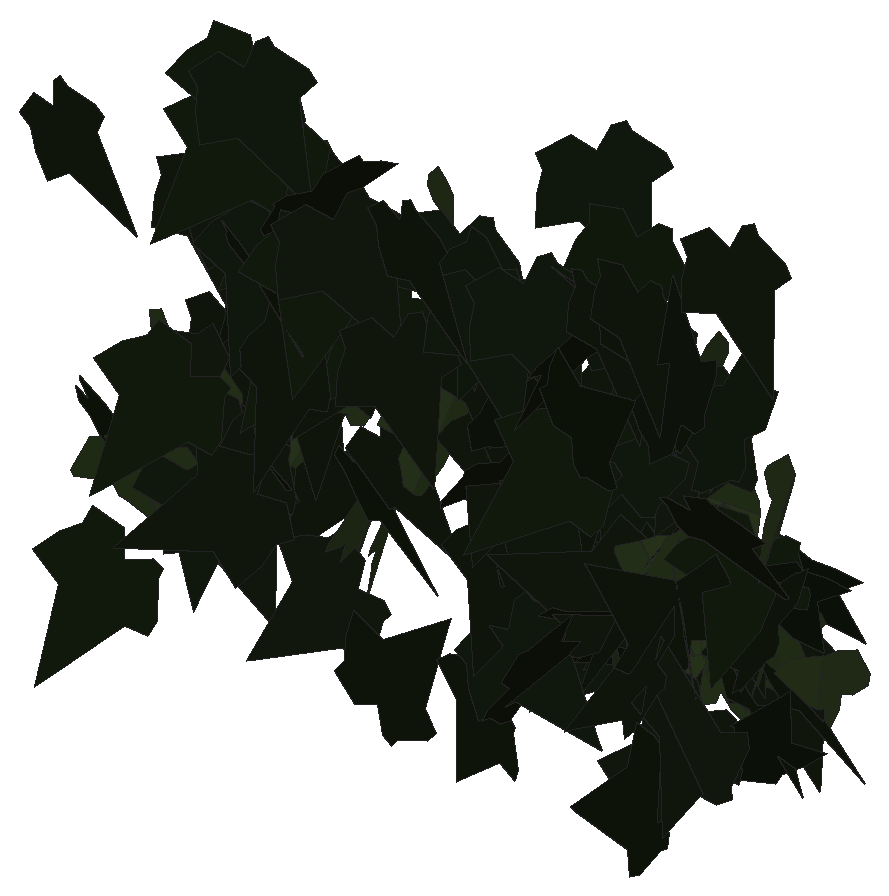
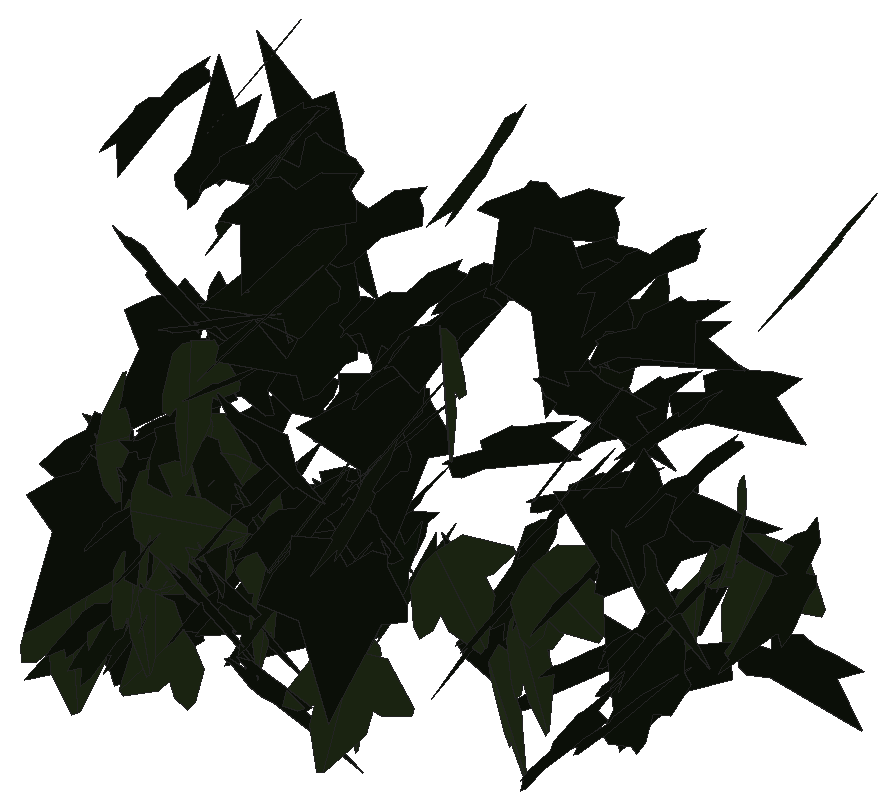
# SketchUp Ruby script. Lengths in inches.
U = 1.inch
M = Sketchup.active_model
def pt(a) = Geom::Point3d.new(a.map { |v| v * U })
def face(e, loops, mat)
  f = e.add_face(loops[0].map { |a| pt(a) })
  loops[1..].each { |l| e.add_face(l.map { |a| pt(a) }).erase! }
  f.material = f.back_material = mat if mat
  f
end
# faces: each face lists its corners as indices into pts; further lists are holes
def faces(e, pts, list, mat = nil) = list.each { |f| face(e, (f[0].is_a?(Array) ? f : [f]).map { |l| l.map { |i| pts[i] } }, mat) }
# xy, xz, yz: faces in a plane at the given z, y or x. An outline is a flat list of corners, or four numbers for a rectangle; further outlines are holes
def ring(l) = l.size == 4 ? [[l[0], l[1]], [l[2], l[1]], [l[2], l[3]], [l[0], l[3]]] : l.each_slice(2).to_a
def flat(e, list, mat, &to3) = list.each { |f| face(e, (f[0].is_a?(Array) ? f : [f]).map { |l| ring(l).map { |u, v| to3.(u, v) } }, mat) }
def xy(e, z, list, mat = nil) = flat(e, list, mat) { |x, y| [x, y, z] }
def xz(e, y, list, mat = nil) = flat(e, list, mat) { |x, z| [x, y, z] }
def yz(e, x, list, mat = nil) = flat(e, list, mat) { |y, z| [x, y, z] }
def lines(e, pts, list) = list.each { |a, b| e.add_line(pt(pts[a]), pt(pts[b])) }
# prism: a flat outline (further loops are holes) pulled along v
def prism(e, loops, v, mat = nil)
  f = face(e, loops, mat); d = Geom::Vector3d.new(v.map { |x| x * U })
  f.pushpull(f.normal.samedirection?(d) ? d.length : -d.length)
end
def box(e, o, s, mat = nil) = prism(e, [[o, [o[0] + s[0], o[1], o[2]], [o[0] + s[0], o[1] + s[1], o[2]], [o[0], o[1] + s[1], o[2]]]], [0, 0, s[2]], mat)
def at(x, y, z, deg = 0) = Geom::Transformation.translation(pt([x, y, z])) * Geom::Transformation.rotation(ORIGIN, Z_AXIS, deg.degrees)
def axes(o, x, y, z) = Geom::Transformation.new([*x, 0, *y, 0, *z, 0, *pt(o).to_a, 1])
def part(name) = M.definitions.add(name)
# library, detail: a bought-in or finely detailed component or shape, given as its bounding box
def library(name, o, s) = part(name).tap { |d| box(d.entities, o, s) }
def detail(e, o, s) = box(e.add_group.entities, o, s)
def put(e, d, t, mat = nil) = e.add_instance(d, t).tap { |i| i.material = mat if mat }
def group(e, t, mat = nil) = e.add_group.tap { |g| g.transformation = t; g.material = mat if mat }.entities
root = M.entities
M.materials.add("efeu1").color = [18, 25, 13]
M.materials.add("efeu2").color = [43, 57, 29]
c1 = part("ivyleaf_9")
p = [[1.54,2.16,1.25],[1.36,2.04,1.19],[-0.21,0.99,0.68],[-0.71,1.11,0.82],[-0.85,0.86,0.67],[-0.8,0.17,0.21],
  [-0.9,-0.01,0.1],[-0.67,-0.16,-0.02],[-0.08,-0.08,-0.05],[-0.03,-0.6,-0.4],[0.65,-0.88,-0.66],[0.83,-0.6,-0.49],
  [1.29,-0.42,-0.43],[1.8125,-0.07,-0.26],[1.21,0.44,0.15]]
faces(c1.entities,p,[[0,1,2,3,4,5,6,7,8,9,10,11,12,13,14]],"efeu1")
c2 = part("ivyleaf_10")
p = [[0,0.5,-0.03],[-0.0625,2.02,-0.43],[-0.19,2.01,-0.46],[-0.54,1.05,-0.29],[-0.52,0.625,-0.18],[-0.83,0.76,-0.28],
  [-1.16,0.64,-0.33],[-1.15,0.33,-0.24],[-0.77,-0.39,0.02],[-0.3,-0.51,0.16],[0.04,-0.48,0.23],[-0.02,2.01,-0.4375],
  [-0.06,2.01,-0.43],[0.04,-0.49,0.23],[0.67,-0.49,0.14],[1.38,0.36,-0.2],[1.375,0.51,-0.24],[0.81,0.65,-0.19],
  [0.62,0.59,-0.15],[0.6,1.09,-0.28],[0.5,1.23,-0.31]]
faces(c2.entities,p,[[0,1,2,3,4,5,6,7,8,9,10],[11,12,0,13,14,15,16,17,18,19,20]],"efeu2")
put(root,c1,axes([37.94,218.92,253.93],[0.31107,-0.3532,-0.16877],[-0.06359,0.16711,-0.46694],[0.38626,0.31196,0.05905]))
put(root,c1,axes([37.98,219.44,250.43],[0.43291,-0.22548,-0.10839],[-0.09049,0.06083,-0.48797],[0.23324,0.44211,0.01186]))
put(root,c1,axes([38.08,221.1,252.23],[0.08499,-0.48929,-0.05807],[0.02582,0.06327,-0.49531],[0.49205,0.0812,0.03603]))
put(root,c1,axes([38.19,221.3,250.65],[0.18802,-0.45638,-0.07977],[-0.02468,0.0761,-0.49356],[0.46264,0.18954,0.00609]))
put(root,c1,axes([38.63,221.29,251.3125],[-0.40733,0.25168,-0.14401],[0.11208,-0.09236,-0.47844],[-0.26743,-0.42205,0.01883]))
put(root,c2,axes([38.38,219.93,251.125],[-0.20143,0.40317,-0.21651],[0.07165,-0.20586,-0.44999],[-0.45199,-0.21231,0.02516]))
put(root,c1,axes([38.6875,218.96,249.12],[-0.45267,-0.21002,-0.0313],[0.029,0.01186,-0.49902],[0.21035,-0.4536,0.00144]))
put(root,c2,axes([38.6,219.23,250.24],[-0.4384,-0.19936,-0.13439],[0.11846,0.06411,-0.48152],[0.20922,-0.45403,-0.00898]))
put(root,c2,axes([38.61,220.32,250.48],[-0.06607,0.477,-0.13456],[0.01467,-0.13381,-0.48154],[-0.4954,-0.06758,0.00369]))
put(root,c1,axes([38.65,221.11,253.67],[-0.21464,-0.44733,0.06182],[-0.00726,-0.06502,-0.4957],[0.45153,-0.2137,0.02141]))
put(root,c1,axes([38.33,221.52,251.59],[0.24057,-0.21984,0.3792],[0.28084,-0.2548,-0.32589],[0.33653,0.36979,0.00089]))
put(root,c1,axes([38.55,220.71,252.5],[0.26925,-0.33348,-0.25747],[-0.01902,0.29563,-0.40279],[0.42088,0.2267,0.14651]))
put(root,c1,axes([38.76,221.4,249.4],[-0.16154,-0.40828,0.23918],[0.0026,-0.2535,-0.43097],[0.47318,-0.138,0.08402]))
put(root,c1,axes([38.97,220.6875,253.22],[-0.36194,-0.31409,0.14265],[-0.07413,-0.13111,-0.47678],[0.3369,-0.36628,0.04834]))
put(root,c1,axes([39.17,219.76,250.9],[-0.4859,-0.00921,0.11755],[-0.11753,-0.00238,-0.48598],[0.00951,-0.49991,0.00015]))
put(root,c1,axes([38.56,221.06,249.46],[0.06355,-0.2335,0.43754],[0.27744,-0.3489,-0.22649],[0.41108,0.27157,0.08522]))
put(root,c1,axes([38.93,220.3,249.48],[-0.0009,-0.42571,-0.26223],[0.04803,0.26095,-0.42379],[0.49769,-0.02595,0.04042]))
put(root,c1,axes([39.09,221.9,249.2],[-0.08746,-0.40199,0.28418],[-0.03472,-0.28287,-0.41083],[0.49107,-0.0916,0.02157]))
put(root,c1,axes([39.13,220.49,249.93],[-0.11468,-0.45361,0.17632],[-0.02204,-0.17613,-0.46743],[0.48617,-0.11498,0.02041]))
put(root,c1,axes([38.99,221.59,252.53],[0.22043,-0.44736,-0.03585],[-0.01789,0.03115,-0.49871],[0.44843,0.22114,-0.00227]))
put(root,c1,axes([39.1,219.81,249.96],[-0.04756,-0.49632,0.03742],[0.00435,-0.038,-0.49853],[0.49771,-0.04709,0.00793]))
put(root,c1,axes([39.04,220.5,254.05],[0.10646,-0.42962,-0.23258],[0.0347,0.24409,-0.43499],[0.4873,0.07647,0.08179]))
put(root,c1,axes([39.46,221.11,252.71],[-0.48139,-0.13469,0.01123],[-0.00951,-0.0077,-0.49985],[0.13482,-0.48146,0.00485]))
put(root,c1,axes([39.36,220.53,252.23],[-0.13388,-0.46702,0.11818],[-0.00787,-0.12053,-0.48519],[0.48168,-0.13177,0.02492]))
put(root,c1,axes([39.64,218.79,251.59],[-0.36767,-0.32625,0.09154],[-0.07677,-0.05137,-0.49139],[0.33004,-0.37539,-0.01232]))
put(root,c1,axes([39.34,221.17,250.65],[0.05622,-0.48751,0.0958],[0.01464,-0.09475,-0.49072],[0.49661,0.05798,0.00362]))
put(root,c2,axes([39.66,221.27,250.56],[-0.18255,-0.3388,0.3192],[0.00515,-0.34432,-0.36252],[0.46546,-0.12907,0.1292]))
put(root,c1,axes([39.71,220.84,251.375],[-0.31245,-0.36813,0.12982],[0.01201,-0.17527,-0.46812],[0.39017,-0.28941,0.11837]))
put(root,c1,axes([40.02,219.35,250.17],[-0.03955,-0.18419,-0.46315],[-0.0133,-0.46405,0.18568],[-0.49826,0.02701,0.03181]))
put(root,c1,axes([39.85,221.01,251.1],[-0.08184,-0.3862,0.30684],[-0.02083,-0.30805,-0.39328],[0.49282,-0.07716,0.03434]))
put(root,c1,axes([39.78,219.77,252.4],[0.14237,-0.32323,0.35391],[0.20636,-0.29189,-0.34959],[0.43261,0.24561,0.05029]))
put(root,c1,axes([40.19,220.125,253.3],[0.1405,0.47912,0.02647],[0.00961,0.02477,-0.49929],[-0.47976,0.14081,-0.00225]))
put(root,c2,axes([40.18,221.35,249.28],[0.24768,-0.43322,0.03116],[0.01107,-0.02957,-0.499],[0.4342,0.24788,-0.00506]))
put(root,c2,axes([40.29,220.84,249.54],[0.11401,-0.48629,0.02298],[-0.00139,-0.02393,-0.49943],[0.48683,0.11382,-0.00681]))
put(root,c1,axes([40.42,220.43,248.78],[-0.28231,-0.27839,0.30463],[-0.10902,-0.30567,-0.38037],[0.39801,-0.28119,0.11189]))
put(root,c1,axes([40.43,219.54,251.86],[-0.43205,-0.05215,-0.24619],[0.24228,0.04612,-0.43494],[0.06808,-0.49513,-0.01458]))
put(root,c1,axes([40.49,221.18,251.71],[-0.31409,-0.35015,0.16955],[-0.05255,-0.17773,-0.46438],[0.38547,-0.30953,0.07484]))
put(root,c1,axes([40.28,221.1,250.09],[0.28149,-0.3472,-0.22409],[-0.09424,0.21005,-0.44384],[0.40235,0.29211,0.05281]))
put(root,c2,axes([40.71,221.52,250.4],[-0.15062,-0.42481,0.21646],[0.01978,-0.23238,-0.44228],[0.47636,-0.12466,0.08681]))
put(root,c1,axes([40.4375,220.5,250.12],[0.39536,-0.30238,-0.04748],[-0.03622,0.03081,-0.49773],[0.30394,0.39701,0.00246]))
put(root,c2,axes([40.81,221.4,252.75],[0.33334,-0.30971,-0.20729],[-0.06296,0.22732,-0.44087],[0.36732,0.32001,0.11255]))
put(root,c1,axes([40.74,219.66,253],[-0.2313,-0.44035,-0.05088],[0.0258,0.04392,-0.4974],[0.44253,-0.23272,0.00241]))
put(root,c1,axes([41.01,219.4375,253.51],[-0.05242,-0.3479,-0.35527],[0.1452,0.33096,-0.34552],[0.47557,-0.13939,0.06633]))
put(root,c1,axes([41.28,221.03,252.73],[-0.00397,-0.49095,-0.09464],[0.00418,0.0946,-0.49095],[0.49997,-0.00469,0.00335]))
put(root,c1,axes([41.4375,219.59,248.28],[-0.18447,0.11953,0.44909],[0.34298,-0.29102,0.21834],[0.31359,0.38861,0.02538]))
put(root,c1,axes([41.51,221.73,251.1],[0.35378,-0.32628,-0.1356],[-0.09822,0.09351,-0.48126],[0.33941,0.36715,0.00207]))
put(root,c1,axes([41.78,221.77,250.15],[0.31682,0.32271,-0.21326],[-0.15115,-0.15047,-0.45223],[-0.35606,0.35102,0.00221]))
put(root,c1,axes([41.64,221.24,252.29],[-0.07125,-0.4399,0.22675],[-0.02798,-0.22514,-0.44557],[0.49411,-0.07618,0.00746]))
put(root,c1,axes([41.6,220.97,251.55],[0.15039,-0.47232,0.06552],[0.01618,-0.0636,-0.49567],[0.47657,0.15121,-0.00385]))
put(root,c1,axes([41.77,219.4,252.47],[0.04234,-0.45452,-0.20401],[-0.01739,0.20327,-0.45648],[0.4979,0.04575,0.00141]))
put(root,c2,axes([41.92,221.55,248.84],[-0.35045,-0.34055,-0.1059],[0.12979,0.0165,-0.48258],[0.33217,-0.36573,0.07684]))
put(root,c1,axes([41.73,221.2,249.53],[0.01049,-0.23126,0.44318],[0.10511,-0.43235,-0.2281],[0.48871,0.09795,0.03954]))
put(root,c1,axes([41.79,219.51,253.74],[0.29994,-0.39767,-0.0435],[-0.02218,0.03775,-0.49808],[0.39943,0.30072,0.00501]))
put(root,c1,axes([42.03,220.51,252.59],[0.02693,-0.47627,-0.14979],[0.01673,0.15079,-0.47643],[0.49899,0.02065,0.02406]))
put(root,c1,axes([42.15,220.49,251.04],[0.04594,0.07772,0.49178],[0.28341,0.40197,-0.09],[-0.40935,0.28702,-0.00712]))
put(root,c1,axes([42.16,220.66,250.82],[-0.07819,-0.43823,0.22769],[0.0357,-0.23494,-0.43992],[0.49256,-0.05254,0.06802]))
put(root,c2,axes([42.39,220.97,248.75],[0.15018,-0.46691,-0.09714],[-0.0137,0.09758,-0.49019],[0.47672,0.1499,0.01652]))
put(root,c1,axes([42.48,220.18,251.04],[0.07405,0.4903,-0.06422],[-0.01235,-0.06308,-0.49585],[-0.49433,0.07502,0.00276]))
put(root,c1,axes([42.78,221.86,251.26],[-0.46361,0.08666,-0.16601],[-0.16675,0.01069,0.47125],[0.08522,0.49232,0.01899]))
put(root,c1,axes([42.52,220.83,250.17],[-0.43007,-0.07254,-0.24449],[0.23876,0.05394,-0.43599],[0.08963,-0.49176,-0.01176]))
put(root,c1,axes([42.3,221.67,250.53],[0.09053,-0.44675,0.20548],[0.03452,-0.20264,-0.45579],[0.49052,0.09671,-0.00585]))
put(root,c1,axes([42.4,220.36,249.79],[-0.04837,-0.42669,0.25611],[0.021,-0.25884,-0.42727],[0.49721,-0.03058,0.04296]))
put(root,c1,axes([42.86,221.82,248.65],[-0.49701,0.05229,0.01578],[-0.01814,-0.02179,-0.4992],[-0.05152,-0.49678,0.02356]))
put(root,c1,axes([42.59,221.5,250.4375],[0.02454,-0.48577,-0.11588],[-0.01917,0.11502,-0.48621],[0.49903,0.02831,-0.01298]))
put(root,c1,axes([42.625,221.5,253.9375],[-0.03978,-0.38436,-0.31731],[0.02871,0.31602,-0.3864],[0.49759,-0.04896,-0.00307]))
put(root,c1,axes([42.69,219.72,248.6],[-0.03846,-0.3218,0.38075],[0.04099,-0.38262,-0.31925],[0.49683,0.00666,0.05581]))
put(root,c1,axes([42.54,221,252.29],[0.4445,-0.09124,0.20998],[0.21325,-0.00187,-0.45224],[0.08331,0.4916,0.03725]))
put(root,c1,axes([42.79,220.17,253.1],[0.0414,-0.4169,-0.27291],[0.0221,0.27512,-0.41692],[0.49779,0.02246,0.04121]))
put(root,c1,axes([42.81,220.43,249.125],[0.39281,0.23918,0.1962],[0.15348,0.12465,-0.45924],[-0.2686,0.42102,0.0245]))
put(root,c2,axes([43.23,221.14,249.26],[-0.02012,0.28396,0.41105],[-0.30831,0.31664,-0.23384],[-0.39311,-0.26287,0.16235]))
put(root,c1,axes([42.87,219.85,249.4],[0.13387,-0.34009,-0.3412],[0.01466,0.35684,-0.34993],[0.48152,0.08368,0.10551]))
put(root,c1,axes([42.8,220.88,252.77],[0.44337,-0.16788,0.15886],[0.16343,-0.01528,-0.47229],[0.16343,0.47073,0.04132]))
put(root,c1,axes([42.9,221.46,249.51],[0.37591,-0.32624,0.0475],[0.03386,-0.03346,-0.49773],[0.32794,0.37742,-0.00306]))
put(root,c1,axes([42.98,221.33,252.48],[0.25539,-0.40389,-0.14714],[0.0038,0.17326,-0.46901],[0.42984,0.23844,0.09156]))
put(root,c1,axes([43.54,220.79,249.56],[-0.09442,0.0014,0.491],[-0.4746,-0.12844,-0.0909],[0.12587,-0.48322,0.02558]))
put(root,c1,axes([43.22,219.4375,249.14],[0.13256,0.30793,0.37095],[0.14811,0.3401,-0.33525],[-0.45879,0.19876,-0.00104]))
put(root,c1,axes([43.08,221.61,250.35],[0.17836,-0.44868,-0.12989],[-0.02398,0.13006,-0.48219],[0.46649,0.17824,0.02487]))
put(root,c1,axes([43.53,221.7,249.45],[-0.49364,0.07894,-0.00924],[0.00893,-0.0027,-0.49991],[-0.07898,-0.49372,0.00126]))
put(root,c1,axes([43.5625,222.02,249.53],[-0.48564,0.085,-0.08321],[0.07968,-0.0272,-0.49286],[-0.08832,-0.49197,0.01288]))
put(root,c1,axes([43.625,219.96,251.59],[-0.43378,-0.21509,0.12477],[-0.11088,-0.05726,-0.48418],[0.22257,-0.44773,0.00198]))
put(root,c2,axes([43.88,222.06,250.21],[-0.02316,-0.00217,-0.49946],[-0.49681,0.05153,0.02281],[0.05137,0.49733,-0.00455]))
put(root,c1,axes([43.84,220.95,251.48],[0.00031,-0.00738,0.49995],[-0.31608,0.38737,0.00591],[-0.38742,-0.31605,-0.00442]))
put(root,c2,axes([43.64,221.8,251.77],[-0.00128,-0.47737,-0.14872],[0.02093,0.14854,-0.47697],[0.49956,-0.00745,0.0196]))
put(root,c1,axes([43.79,219.91,253.0625],[-0.19251,0.38025,-0.26144],[0.05351,-0.26298,-0.42188],[-0.45834,-0.19041,0.06056]))
put(root,c1,axes([43.71,220.89,249.96],[-0.41836,0.1111,-0.25026],[0.22951,-0.10694,-0.43115],[-0.14933,-0.47563,0.03849]))
put(root,c1,axes([43.67,220.57,251.02],[-0.44275,0.05913,0.22467],[0.21334,-0.08793,0.44357],[0.09197,0.48864,0.05263]))
put(root,c1,axes([43.51,221.54,249.26],[0.10267,-0.48899,0.01876],[0.00032,-0.0191,-0.49964],[0.48935,0.1026,-0.00361]))
put(root,c1,axes([43.9375,221.39,250.52],[-0.14363,0.47573,0.05523],[-0.02361,0.05055,-0.49688],[-0.47835,-0.14534,0.00794]))
put(root,c1,axes([43.8,221.43,252.05],[-0.3938,-0.27471,0.13948],[0.00813,-0.23555,-0.44096],[0.30799,-0.34503,0.18999]))
put(root,c1,axes([43.83,221.79,251.25],[-0.19278,-0.42279,0.18461],[0.01937,-0.20732,-0.45458],[0.46093,-0.16812,0.09631]))
put(root,c1,axes([43.77,220.67,253.74],[-0.03378,-0.49875,0.0103],[0.00167,-0.01044,-0.49989],[0.49886,-0.03373,0.00237]))
put(root,c2,axes([43.79,220.93,250.07],[-0.43798,-0.13487,-0.19996],[0.22294,-0.06817,-0.44233],[0.09205,-0.47662,0.11984]))
put(root,c2,axes([43.91,221.45,250.57],[0.26642,-0.40402,0.12564],[0.0658,-0.1071,-0.48394],[0.41796,0.2744,-0.0039]))
put(root,c2,axes([44.01,221.17,249.47],[0.13471,0.46505,-0.12481],[-0.0971,-0.1007,-0.48003],[-0.47162,0.15357,0.06319]))
put(root,c1,axes([43.89,220.18,253.32],[0.13552,-0.47871,0.04972],[0.01891,-0.04632,-0.49749],[0.48091,0.13672,0.00555]))
put(root,c2,axes([43.84,221.82,248.67],[0.35128,-0.1222,0.33417],[0.35528,0.09485,-0.33879],[0.01941,0.47547,0.15347]))
put(root,c1,axes([43.93,220.49,253.05],[0.19933,-0.45288,0.07185],[0.02982,-0.06537,-0.49481],[0.45758,0.20155,0.00095]))
put(root,c2,axes([44.23,221.9,249.78],[-0.38889,0.31114,0.04426],[-0.05601,0.00067,-0.49685],[-0.30924,-0.3914,0.03433]))
put(root,c1,axes([43.98,221.76,249.86],[0.16919,-0.46767,-0.05157],[-0.00594,0.05268,-0.49718],[0.47047,0.16885,0.01227]))
put(root,c2,axes([44.27,221.88,249.3125],[0.03067,-0.49831,-0.02732],[-0.00094,0.02732,-0.49925],[0.49906,0.03068,0.00074]))
put(root,c1,axes([44.5,220.02,249.56],[-0.42626,0.26051,0.02081],[-0.01781,0.01077,-0.49957],[-0.26073,-0.42664,0.0001]))
put(root,c2,axes([44.24,221.04,250.4375],[-0.14294,-0.46057,-0.13208],[0.0948,0.10792,-0.47892],[0.46966,-0.16195,0.05647]))
put(root,c1,axes([44.48,220.58,249.63],[0.09855,0.05997,0.48651],[-0.44598,-0.19499,0.11437],[0.20345,-0.45649,0.01506]))
put(root,c1,axes([44.33,221.79,250.02],[-0.03199,-0.49623,0.05227],[0.00602,-0.05276,-0.49717],[0.49894,-0.03118,0.00935]))
put(root,c1,axes([44.96,220.8,251.93],[-0.24932,0.25142,0.35303],[-0.27784,0.21986,-0.3528],[-0.33264,-0.37209,0.03008]))
put(root,c1,axes([44.33,221.65,248.83],[0.29416,-0.40284,0.03452],[0.01389,-0.0326,-0.49874],[0.40408,0.29437,-0.00799]))
put(root,c2,axes([44.64,221.61,249.29],[-0.26498,-0.389,-0.16871],[0.09529,0.13923,-0.47068],[0.41316,-0.2816,0.00035]))
put(root,c1,axes([44.36,218.96,252.55],[-0.05509,0.0466,0.49477],[0.30635,-0.38877,0.07073],[0.39129,0.31094,0.01428]))
put(root,c2,axes([44.72,221.54,249.42],[0.32084,-0.38212,-0.03232],[-0.02166,0.02402,-0.49895],[0.38287,0.32157,-0.00114]))
put(root,c1,axes([44.56,221.84,249.85],[0.44739,0.22324,0.00304],[0.00207,0.00267,-0.49999],[-0.22325,0.44739,0.00147]))
put(root,c1,axes([44.53,222,248.92],[0.09257,-0.46866,-0.14761],[-0.0266,0.14521,-0.47771],[0.49064,0.09629,0.00195]))
put(root,c1,axes([44.53,219.75,253.8],[0.13504,-0.47233,0.09309],[0.02632,-0.0893,-0.49126],[0.4807,0.13757,0.00074]))
put(root,c2,axes([44.59,221.93,250.65],[0.08752,-0.16535,0.46368],[0.28465,-0.36724,-0.18469],[0.40164,0.2963,0.02985]))
put(root,c1,axes([44.74,221.31,250.37],[-0.24522,-0.43573,-0.00219],[0.05082,-0.0261,-0.49672],[0.43276,-0.24384,0.05709]))
put(root,c1,axes([44.52,221.89,248.77],[0.40414,-0.2944,-0.00019],[0.02112,0.02932,-0.49869],[0.29364,0.40308,0.03613]))
put(root,c2,axes([44.94,222.07,248.73],[-0.24513,-0.43551,0.01569],[0.00455,-0.02055,-0.49956],[0.43576,-0.24477,0.01404]))
put(root,c1,axes([44.82,221.24,250.05],[0.36925,0.33504,-0.03751],[-0.0252,-0.02804,-0.49858],[-0.33619,0.37009,-0.00382]))
put(root,c1,axes([44.72,220.25,249.81],[-0.06907,0.03776,0.49376],[0.0766,-0.49173,0.04832],[0.48925,0.08232,0.06214]))
put(root,c1,axes([44.68,220.46,251.125],[0.49774,0.04591,-0.01218],[-0.01216,-0.00083,-0.49985],[-0.04592,0.49789,0.00029]))
put(root,c1,axes([44.93,219.53,248.33],[-0.0621,-0.06692,0.49159],[-0.21487,-0.44293,-0.08744],[0.44718,-0.22212,0.02625]))
put(root,c1,axes([45.07,219.85,248.5],[-0.4043,-0.2389,0.17165],[0.15263,0.07905,0.46953],[-0.25148,0.43206,0.00901]))
put(root,c1,axes([44.8125,220.38,248.95],[-0.0616,-0.45131,0.20621],[-0.01437,-0.20608,-0.45533],[0.49598,-0.06202,0.01242]))
put(root,c1,axes([44.7,221.02,248.1],[0.41803,0.26603,0.06695],[-0.05792,-0.03367,0.49549],[0.26814,-0.42201,0.00266]))
put(root,c1,axes([45.02,219.79,252.61],[-0.05363,-0.39326,0.30409],[0.19704,0.26398,0.37615],[-0.4564,0.16018,0.12666]))
put(root,c1,axes([45.33,220.88,249.92],[-0.33536,0.3502,0.12204],[-0.09515,0.07778,-0.48466],[-0.35844,-0.34829,0.01448]))
put(root,c1,axes([44.83,220.82,253.92],[0.12102,-0.46504,-0.13817],[-0.02656,0.13584,-0.48046],[0.48441,0.12363,0.00817]))
